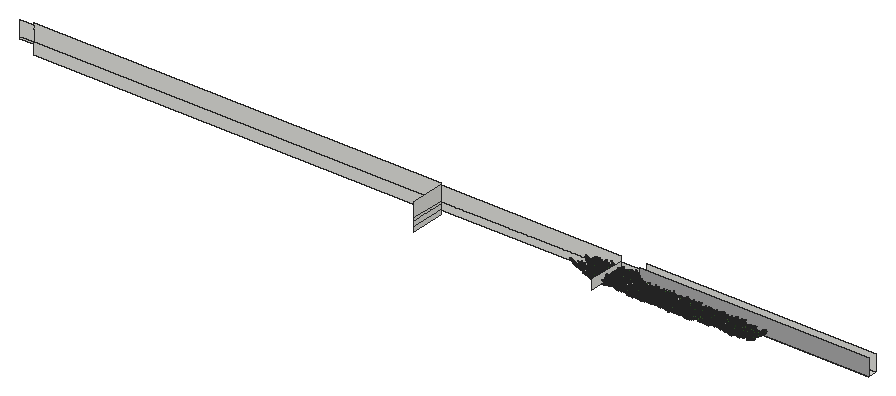
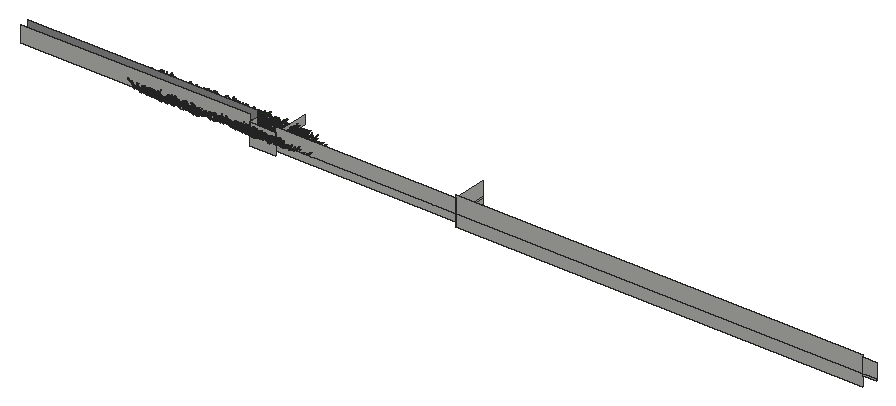
# SketchUp Ruby script. Lengths in inches.
U = 1.inch
M = Sketchup.active_model
def pt(a) = Geom::Point3d.new(a.map { |v| v * U })
def face(e, loops, mat)
  f = e.add_face(loops[0].map { |a| pt(a) })
  loops[1..].each { |l| e.add_face(l.map { |a| pt(a) }).erase! }
  f.material = f.back_material = mat if mat
  f
end
# faces: each face lists its corners as indices into pts; further lists are holes
def faces(e, pts, list, mat = nil) = list.each { |f| face(e, (f[0].is_a?(Array) ? f : [f]).map { |l| l.map { |i| pts[i] } }, mat) }
# xy, xz, yz: faces in a plane at the given z, y or x. An outline is a flat list of corners, or four numbers for a rectangle; further outlines are holes
def ring(l) = l.size == 4 ? [[l[0], l[1]], [l[2], l[1]], [l[2], l[3]], [l[0], l[3]]] : l.each_slice(2).to_a
def flat(e, list, mat, &to3) = list.each { |f| face(e, (f[0].is_a?(Array) ? f : [f]).map { |l| ring(l).map { |u, v| to3.(u, v) } }, mat) }
def xy(e, z, list, mat = nil) = flat(e, list, mat) { |x, y| [x, y, z] }
def xz(e, y, list, mat = nil) = flat(e, list, mat) { |x, z| [x, y, z] }
def yz(e, x, list, mat = nil) = flat(e, list, mat) { |y, z| [x, y, z] }
def lines(e, pts, list) = list.each { |a, b| e.add_line(pt(pts[a]), pt(pts[b])) }
# prism: a flat outline (further loops are holes) pulled along v
def prism(e, loops, v, mat = nil)
  f = face(e, loops, mat); d = Geom::Vector3d.new(v.map { |x| x * U })
  f.pushpull(f.normal.samedirection?(d) ? d.length : -d.length)
end
def box(e, o, s, mat = nil) = prism(e, [[o, [o[0] + s[0], o[1], o[2]], [o[0] + s[0], o[1] + s[1], o[2]], [o[0], o[1] + s[1], o[2]]]], [0, 0, s[2]], mat)
def at(x, y, z, deg = 0) = Geom::Transformation.translation(pt([x, y, z])) * Geom::Transformation.rotation(ORIGIN, Z_AXIS, deg.degrees)
def axes(o, x, y, z) = Geom::Transformation.new([*x, 0, *y, 0, *z, 0, *pt(o).to_a, 1])
def part(name) = M.definitions.add(name)
# library, detail: a bought-in or finely detailed component or shape, given as its bounding box
def library(name, o, s) = part(name).tap { |d| box(d.entities, o, s) }
def detail(e, o, s) = box(e.add_group.entities, o, s)
def put(e, d, t, mat = nil) = e.add_instance(d, t).tap { |i| i.material = mat if mat }
def group(e, t, mat = nil) = e.add_group.tap { |g| g.transformation = t; g.material = mat if mat }.entities
root = M.entities
M.materials.add("Material82").color = [68, 110, 58]
M.materials.add("Material83").color = [48, 90, 38]
M.materials.add("Material84").color = [68, 110, 48]
M.materials.add("Material85").color = [48, 90, 48]
M.materials.add("Material86").color = [58, 110, 58]
M.materials.add("Material87").color = [58, 90, 38]
M.materials.add("Material88").color = [68, 100, 58]
M.materials.add("Material89").color = [48, 100, 38]
M.materials.add("[Color M03]1").color = [170, 170, 170]
c1 = part("grass00")
p = [[-0.6875,0.15,0],[-0.56,0.08,5.52],[-0.04,0.03,2.76],[0.48,-0.02,0],[0.35,-0.02,5.52],[-0.1,-0.14,5.52],
  [-0.12,0.65,8.37],[-0.42,0.65,8.37]]
faces(c1.entities,p,[[0,1,2,3],[3,2,4],[1,5,2],[5,4,2],[1,6,5],[4,5,6],[7,6,1]])
c2 = part("Group16\#1")
put(c2.entities,c1,axes([1.44,-0.61,-0.01],[0.05352,0.12609,0],[-0.10704,0.04543,0.07239],[0.06664,-0.02828,0.11628]),"Material85")
put(c2.entities,c1,axes([0.76,-0.15,-0.01],[0.04676,0.24062,0],[-0.23162,0.04501,0.06642],[0.0652,-0.01267,0.23595]),"Material82")
put(c2.entities,c1,axes([0.79,0.01,-0.01],[-0.00606,0.34651,0],[-0.34381,-0.00602,0.0432],[0.04319,0.00076,0.34386]))
put(c2.entities,c1,axes([1,0.23,-0.01],[-0.07192,0.31144,0],[-0.28722,-0.06632,0.1236],[0.12043,0.02781,0.29478]),"Material84")
put(c2.entities,c1,axes([1.66,0.77,-0.01],[-0.13828,0.29651,0],[-0.21551,-0.1005,0.22471],[0.20365,0.09498,0.23779]),"Material89")
put(c2.entities,c1,axes([0.6875,0.52,-0.01],[-0.18126,0.24051,0],[-0.22746,-0.17142,0.09788],[0.07817,0.05891,0.28481]),"Material84")
put(c2.entities,c1,axes([0.68,0.78,-0.01],[-0.215,0.18688,0],[-0.12385,-0.14248,0.21334],[0.13995,0.16101,0.18878]),"Material82")
put(c2.entities,c1,axes([0.56,1,-0.01],[-0.13756,0.07624,0],[-0.06159,-0.11112,0.0927],[0.04494,0.08108,0.12705]),"Material84")
put(c2.entities,c1,axes([0.2,0.64,-0.01],[-0.23729,0.07254,0],[-0.05711,-0.18681,0.153],[0.04473,0.14632,0.19535]),"Material89")
put(c2.entities,c1,axes([0.0625,0.72,-0.01],[-0.28874,0.02525,0],[-0.02179,-0.24916,0.14647],[0.01276,0.14591,0.25012]),"Material82")
put(c2.entities,c1,axes([-0.08,0.62,-0.01],[-0.34089,-0.04187,0],[0.03255,-0.26504,0.216],[-0.02633,0.21439,0.26703]),"Material89")
put(c2.entities,c1,axes([-0.34,0.98,-0.01],[-0.14314,-0.0493,0],[0.04397,-0.12769,0.06843],[-0.02228,0.0647,0.13505]),"Material89")
put(c2.entities,c1,axes([-0.87,1.45,-0.01],[-0.23488,-0.14114,0],[0.13761,-0.22901,0.06087],[-0.03135,0.05217,0.26717]))
put(c2.entities,c1,axes([-0.72,0.77,-0.01],[-0.14208,-0.13251,0],[0.07209,-0.0773,0.16301],[-0.11118,0.11922,0.1057]),"Material89")
put(c2.entities,c1,axes([-0.62,0.43,-0.01],[-0.14845,-0.21203,0],[0.18654,-0.13061,0.12304],[-0.10079,0.07057,0.22772]),"Material82")
put(c2.entities,c1,axes([-0.68,0.29,-0.01],[-0.13639,-0.32136,0],[0.31723,-0.13464,0.05579],[-0.05136,0.0218,0.34462]),"Material83")
put(c2.entities,c1,axes([-0.64,0.125,-0.01],[-0.0458,-0.23569,0],[0.22124,-0.043,0.08276],[-0.08124,0.01579,0.22538]),"Material86")
put(c2.entities,c1,axes([-1.6,-0.03,-0.01],[0.00576,-0.32897,0],[0.27526,0.00482,0.18018],[-0.18015,-0.00315,0.2753]),"Material84")
put(c2.entities,c1,axes([-1.36,-0.31,-0.01],[0.05718,-0.24765,0],[0.18172,0.04196,0.17267],[-0.16825,-0.03885,0.1865]),"Material89")
put(c2.entities,c1,axes([-1.54,-0.72,-0.01],[0.06537,-0.14017,0],[0.13555,0.06321,0.03939],[-0.0357,-0.01665,0.14956]))
put(c2.entities,c1,axes([-1.19,-0.9,-0.01],[0.09597,-0.12735,0],[0.11214,0.08451,0.07557],[-0.06035,-0.04548,0.14042]),"Material88")
put(c2.entities,c1,axes([-0.47,-0.54,-0.01],[0.11588,-0.10072,0],[0.0618,0.0711,0.12124],[-0.07953,-0.0915,0.0942]))
put(c2.entities,c1,axes([-0.47,-0.84,-0.01],[0.11927,-0.0661,0],[0.06603,0.11913,0.00646],[-0.00313,-0.00565,0.13621]),"Material84")
put(c2.entities,c1,axes([-0.38,-1.24,-0.01],[0.28037,-0.08571,0],[0.0618,0.20215,0.20315],[-0.05939,-0.19428,0.21139]),"Material88")
put(c2.entities,c1,axes([-0.06,-0.66,-0.01],[0.22719,-0.01987,0],[0.01247,0.14255,0.17758],[-0.01547,-0.17691,0.1431]),"Material87")
put(c2.entities,c1,axes([0.11,-0.89,-0.01],[0.14882,0.01828,0],[-0.01058,0.08611,0.12229],[0.01491,-0.12138,0.08676]),"Material85")
put(c2.entities,c1,axes([0.25,-0.72,-0.01],[0.20481,0.07053,0],[-0.06206,0.18022,0.10291],[0.03351,-0.0973,0.1906]),"Material85")
put(c2.entities,c1,axes([0.85,-1.42,-0.01],[0.16481,0.09904,0],[-0.09472,0.15762,0.05616],[0.02893,-0.04814,0.18389]),"Material84")
put(c2.entities,c1,axes([1.01,-1.09,-0.01],[0.21858,0.20385,0],[-0.17495,0.1876,0.15339],[0.10462,-0.11218,0.25652]),"Material89")
put(c2.entities,c1,axes([1.01,-0.71,-0.01],[0.08733,0.12473,0],[-0.06445,0.04512,0.13037],[0.1068,-0.07477,0.07867]),"Material85")
c3 = part("Group15\#1")
put(c3.entities,c2,at(0,0,0))
c4 = part("3darcstudiotree_grass00\#1")
put(c4.entities,c3,at(0,0,0))
xy(root,-34.17,[[626.68,381.72,782.78,387.84]])
xz(root,381.72,[[626.68,-34.17,782.78,-22.8]],"[Color M03]1")
xz(root,387.84,[[208.91,-42.1875,486.41,-34.17],[609.09,-42.1875,626.68,-34.17],[486.41,-39.125,609.09,-34.17],[200.03,-35.625,208.91,-34.17],[200.03,-34.17,208.91,-24.25],
  [208.91,-34.17,486.41,-22.8],[486.41,-34.17,609.09,-24.25],[609.09,-34.17,626.68,-27.66],[626.68,-34.17,782.78,-22.8]])
yz(root,486.41,[[364.46,-42.1875,387.84,-39.125],[364.46,-39.125,387.84,-35.625],[364.46,-35.625,387.84,-34.17],[364.46,-34.17,387.84,-24.25]])
yz(root,609.09,[[362.97,-34.17,387.84,-27.66]])
yz(root,626.68,[[381.72,-34.17,387.84,-27.66]])
put(root,c4,axes([652.09,372.41,-34.17],[-4.26886,-0.01451,0],[0.03771,-1.72573,-0.00939],[0.00047,-0.02147,1.9024]))
put(root,c4,axes([641.22,372.79,-34.17],[3.91894,1.05311,0],[-2.36552,1.3691,-0.06012],[-0.14517,0.08402,1.3502]))
put(root,c4,axes([633.56,373.13,-34.17],[3.33812,-0.00931,0],[0.03014,1.68097,-0.0442],[0.00131,0.07293,1.33678]))
put(root,c4,axes([607.1,373.02,-34.17],[2.55431,1.01117,0],[-3.10398,1.2195,-0.03194],[-0.09397,0.03692,1.36388]))
put(root,c4,axes([664.3125,372.65,-34.17],[-3.78642,0.03695,0],[-0.11198,-1.78455,-0.01248],[-0.00125,-0.01991,1.37214]))
put(root,c4,axes([695.84,372.82,-34.17],[-3.59063,0.36551,0],[-0.927,-1.41632,-0.03018],[-0.05381,-0.08221,1.98332]))
put(root,c4,axes([668.4,372.76,-34.17],[-3.89357,0.61481,0],[-1.50479,-1.48217,-0.00598],[-0.01246,-0.01228,1.70205]))
put(root,c4,axes([631.51,373.3125,-34.17],[-2.43659,-1.39628,0],[3.54139,-0.96116,-0.05298],[0.19991,-0.05426,1.4759]))
put(root,c4,axes([622.52,373.45,-34.17],[2.25035,1.16277,0],[-2.68664,0.80868,-0.04536],[-0.27393,0.08245,1.92466]))
put(root,c4,axes([672.23,374.24,-34.17],[0.94723,-1.59052,0],[4.2139,0.39031,-0.04288],[0.2193,0.02031,1.70449]))
put(root,c4,axes([702.36,374.25,-34.17],[4.40385,0.48107,0],[-1.25638,1.78876,-0.02222],[-0.03253,0.04631,1.93436]))
put(root,c4,axes([664.33,374.63,-34.17],[0.52677,-1.54843,0],[3.37532,0.17859,-0.00096],[0.0064,0.00034,1.71349]))
put(root,c4,axes([607.1,374.65,-34.17],[1.00905,-1.48256,0],[4.12419,0.43657,-0.05256],[0.2523,0.02671,1.59089]))
put(root,c4,axes([669.5,374.45,-34.17],[-2.54975,-1.13663,0],[2.74994,-0.95943,-0.02762],[0.1264,-0.0441,1.68176]))
put(root,c4,axes([655.52,374.86,-34.17],[4.10302,-0.30694,0],[0.8385,1.74326,-0.00778],[0.00611,0.0127,1.42033]))
put(root,c4,axes([628.73,374.0625,-34.17],[-3.06856,1.30795,0],[-2.89535,-1.05647,-0.0352],[-0.142,-0.05181,1.62511]))
put(root,c4,axes([641.16,374.78,-34.17],[0.60137,-1.69863,0],[3.35822,0.18491,-0.0384],[0.22932,0.01263,1.53253]))
put(root,c4,axes([684.16,375.0625,-34.17],[3.06207,-0.55792,0],[1.42852,1.21938,-0.0238],[0.07482,0.06387,1.9133]))
put(root,c4,axes([679.29,374.52,-34.17],[0.41076,1.77313,0],[-3.60416,0.12986,-0.02215],[-0.11578,0.00417,1.42375]))
put(root,c4,axes([623.97,375.43,-34.17],[-0.12471,-1.80139,0],[4.72201,-0.05084,-0.06757],[0.3331,-0.00359,1.74608]))
put(root,c4,axes([633.75,374.875,-34.17],[-0.2328,1.40639,0],[-3.78045,-0.09733,-0.01044],[-0.05523,-0.00142,1.50484]))
put(root,c4,axes([695.93,374.77,-34.17],[-1.9685,1.46825,0],[-4.07305,-0.84931,-0.01892],[-0.07094,-0.01479,1.46501]))
put(root,c4,axes([613.67,375.07,-34.17],[1.86247,1.54763,0],[-3.42195,0.64048,-0.01135],[-0.06523,0.01221,1.80626]))
put(root,c4,axes([602.53,375.22,-34.17],[-0.22309,1.29668,0],[-4.38525,-0.11734,-0.00038],[-0.00168,-0.00004,1.44006]))
put(root,c4,axes([688.73,375.41,-34.17],[1.22817,1.22832,0],[-3.29828,0.51292,-0.04901],[-0.28268,0.04396,1.64754]))
put(root,c4,axes([649.625,375.32,-34.17],[-0.96459,1.39728,0],[-4.50708,-0.48391,-0.06593],[-0.29103,-0.03125,1.60187]))
put(root,c4,axes([647.97,375.42,-34.17],[0.06651,1.49398,0],[-4.62108,0.032,-0.00579],[-0.03066,0.00021,1.83497]))
put(root,c4,axes([616.87,375.59,-34.17],[-3.98386,-0.59662,0],[1.47731,-1.53422,-0.04397],[0.0965,-0.10022,1.92843]))
put(root,c4,axes([644.95,376.5,-34.17],[3.81628,-0.13918,0],[0.37321,1.59155,-0.00914],[0.00528,0.02252,1.90465]))
put(root,c4,axes([616.65,376.41,-34.17],[3.87274,-0.73751,0],[1.55178,1.26734,-0.04306],[0.13654,0.11151,1.95064]))
put(root,c4,axes([694.93,376.96,-34.17],[4.03419,0.29669,0],[-0.75311,1.59264,-0.00417],[-0.00465,0.00984,1.87295]))
put(root,c4,axes([657.29,376.69,-34.17],[1.8424,1.14237,0],[-3.65624,0.91712,-0.00074],[-0.00371,0.00093,1.93092]))
put(root,c4,axes([601.27,376.95,-34.17],[-2.10821,-1.47996,0],[3.50963,-0.77757,-0.0488],[0.18715,-0.04146,1.32723]))
put(root,c4,axes([690.03,376.96,-34.17],[4.26727,0.66803,0],[-1.41698,1.40776,-0.04113],[-0.07249,0.07202,1.37498]))
put(root,c4,axes([672.39,377.2,-34.17],[4.15464,-0.59094,0],[1.53872,1.68251,-0.06016],[0.09162,0.10018,1.52593]))
put(root,c4,axes([668.37,376.61,-34.17],[0.64746,1.71828,0],[-3.59,0.21039,-0.03328],[-0.18561,0.01088,1.53387]))
put(root,c4,axes([606.1,377.25,-34.17],[2.13524,-1.29449,0],[3.0122,0.77275,-0.01966],[0.10051,0.02579,1.64285]))
put(root,c4,axes([641.33,376.78,-34.17],[-1.5249,1.25696,0],[-3.62628,-0.68422,-0.02774],[-0.1175,-0.02217,1.41462]))
put(root,c4,axes([623.77,377.47,-34.17],[3.32502,-0.81851,0],[2.11953,1.33913,-0.03499],[0.11667,0.07371,1.88939]))
put(root,c4,axes([597.38,376.76,-34.17],[-3.35215,0.96429,0],[-2.54913,-1.37823,-0.03459],[-0.11585,-0.06264,1.84283]))
put(root,c4,axes([661.1,377.42,-34.17],[-1.38876,-1.54798,0],[3.56891,-0.49797,-0.03351],[0.18812,-0.02625,1.68972]))
put(root,c4,axes([634.32,376.83,-34.17],[-1.7842,1.38137,0],[-4.14651,-0.83297,-0.01882],[-0.07173,-0.01441,1.49212]))
put(root,c4,axes([680.47,377.7,-34.17],[0.96466,-1.81909,0],[3.32191,0.27398,-0.01603],[0.09156,0.00755,1.48463]))
put(root,c4,axes([614.5,377.27,-34.17],[-2.42169,0.94143,0],[-3.12641,-1.2508,-0.05994],[-0.19111,-0.07646,1.51606]))
put(root,c4,axes([627.52,377.69,-34.17],[-1.63198,-1.29559,0],[3.66951,-0.7189,-0.01655],[0.08632,-0.01691,1.78815]))
put(root,c4,axes([686.3,377.29,-34.17],[-1.97144,1.08801,0],[-3.33394,-0.93955,-0.01309],[-0.05439,-0.01533,1.56859]))
put(root,c4,axes([701.74,377.8,-34.17],[-3.77025,-0.95024,0],[2.35793,-1.45505,-0.05584],[0.17762,-0.10961,1.93872]))
put(root,c4,axes([652.15,377.51,-34.17],[-0.60649,1.78928,0],[-3.60415,-0.19,-0.04319],[-0.29403,-0.0155,1.87209]))
put(root,c4,axes([668.95,378.77,-34.17],[2.12492,-1.52639,0],[3.32667,0.72027,-0.02765],[0.13101,0.02837,1.53783]))
put(root,c4,axes([597.24,378.7,-34.17],[3.10066,0.47843,0],[-1.67535,1.68868,-0.03882],[-0.06401,0.06452,1.55956]))
put(root,c4,axes([602.84,378.47,-34.17],[2.78968,1.01154,0],[-2.64,1.13236,-0.04265],[-0.18761,0.08047,1.90027]))
put(root,c4,axes([612.4,378.8,-34.17],[4.11116,0.47333,0],[-1.05643,1.42708,-0.03197],[-0.04362,0.05892,1.37583]))
put(root,c4,axes([640.57,378.72,-34.17],[3.33503,1.17525,0],[-2.6851,1.18507,-0.00121],[-0.00399,0.00176,1.48985]))
put(root,c4,axes([674.12,379.08,-34.17],[2.11135,-1.17998,0],[3.12805,0.87051,-0.01427],[0.05324,0.01482,1.30992]))
put(root,c4,axes([658.07,379,-34.17],[-2.24585,-1.17679,0],[2.75058,-0.81643,-0.02546],[0.1532,-0.04547,1.94365]))
put(root,c4,axes([679.77,379.3,-34.17],[-1.90322,-1.23489,0],[2.93996,-0.70472,-0.04312],[0.27444,-0.06578,1.92045]))
put(root,c4,axes([606.78,378.9,-34.17],[-2.52665,1.52426,0],[-3.1276,-0.80632,-0.05029],[-0.29899,-0.07708,1.98932]))
put(root,c4,axes([651.6,378.94,-34.17],[-1.50368,1.17097,0],[-3.52829,-0.70467,-0.03106],[-0.12382,-0.02473,1.32443]))
put(root,c4,axes([700.05,379.75,-34.17],[3.38929,-0.88137,0],[2.3631,1.41334,-0.02666],[0.06787,0.04059,1.48784]))
put(root,c4,axes([663.3125,379.73,-34.17],[2.20658,-1.37183,0],[2.86337,0.71632,-0.01781],[0.08885,0.02223,1.50117]))
put(root,c4,axes([645,379.64,-34.17],[0.14571,-1.35454,0],[4.55175,0.07615,-0.04061],[0.20314,0.0034,1.70991]))
put(root,c4,axes([690.06,379.53,-34.17],[3.73542,0.56333,0],[-1.36375,1.40645,-0.02441],[-0.06005,0.06193,1.97124]))
put(root,c4,axes([617.67,379.17,-34.17],[0.11998,1.39847,0],[-4.49149,0.05993,-0.06181],[-0.32467,0.00433,1.77032]))
put(root,c4,axes([685.36,379.47,-34.17],[2.76774,0.7917,0],[-1.93345,1.05126,-0.02439],[-0.09329,0.05072,1.60766]))
put(root,c4,axes([623.83,379.76,-34.17],[2.90846,1.13793,0],[-2.61613,1.03996,-0.02475],[-0.10205,0.04057,1.62992]))
put(root,c4,axes([695.87,379.87,-34.17],[1.66114,1.62878,0],[-3.87747,0.61504,-0.0015],[-0.00686,0.00109,1.54039]))
put(root,c4,axes([627.625,379.91,-34.17],[0.65055,1.72425,0],[-3.43127,0.20135,-0.01524],[-0.11013,0.00646,1.90022]))
put(root,c4,axes([636.29,379.91,-34.17],[-2.50108,0.95556,0],[-2.98511,-1.21518,-0.02879],[-0.10959,-0.04461,1.7592]))
put(root,c4,axes([688.81,380.69,-34.17],[2.03121,-1.05332,0],[3.7313,1.11909,-0.04371],[0.13933,0.04179,1.40723]))
put(root,c4,axes([623.9375,380.76,-34.17],[4.3644,0.14123,0],[-0.27589,1.32601,-0.01884],[-0.00836,0.04017,1.37151]))
put(root,c4,axes([607.96,380.67,-34.17],[4.04964,0.85012,0],[-2.04869,1.51784,-0.02998],[-0.08539,0.06326,1.98098]))
put(root,c4,axes([633.9375,380.75,-34.17],[-0.81871,-1.45227,0],[3.80429,-0.33355,-0.01455],[0.06635,-0.00582,1.36448]))
put(root,c4,axes([669.2,381.01,-34.17],[2.26224,-1.2031,0],[3.43735,1.00525,-0.03781],[0.13632,0.03987,1.4396]))
put(root,c4,axes([653.54,381.18,-34.17],[3.40778,-1.13854,0],[2.78991,1.29874,-0.02128],[0.06823,0.03176,1.60475]))
put(root,c4,axes([673.07,380.76,-34.17],[-4.28344,0.1007,0],[-0.25434,-1.68266,-0.00226],[-0.00079,-0.00521,1.87745]))
put(root,c4,axes([702.07,380.75,-34.17],[-3.53825,1.08299,0],[-2.59336,-1.31776,-0.03049],[-0.10241,-0.05204,1.73706]))
put(root,c4,axes([611.7,381.41,-34.17],[3.8777,-0.38352,0],[0.80355,1.2636,-0.03452],[0.06321,0.0994,1.86367]))
put(root,c4,axes([694.64,381.04,-34.17],[-3.68784,-0.24252,0],[0.55953,-1.32329,-0.01602],[0.01459,-0.0345,1.41148]))
put(root,c4,axes([602.6,381.09,-34.17],[-3.74626,-0.28421,0],[0.67953,-1.39309,-0.01319],[0.01627,-0.03336,1.76124]))
put(root,c4,axes([658.01,381.61,-34.17],[1.48309,-1.18944,0],[3.17184,0.61511,-0.04022],[0.27217,0.05278,1.99791]))
put(root,c4,axes([683.51,381.65,-34.17],[3.41982,0.22152,0],[-0.58321,1.40029,-0.00501],[-0.00425,0.0102,1.40942]))
put(root,c4,axes([616.94,381.62,-34.17],[3.19951,0.37191,0],[-1.24549,1.66647,-0.04213],[-0.05146,0.06886,1.42653]))
put(root,c4,axes([631.55,381.27,-34.17],[1.18703,1.24458,0],[-3.56072,0.52819,-0.04913],[-0.2933,0.04351,1.81865]))
put(root,c4,axes([639.32,381.82,-34.17],[4.2261,-0.33522,0],[0.81524,1.59847,-0.02659],[0.0257,0.05039,1.51897]))
put(root,c4,axes([664.82,381.11,-34.17],[-4.05008,0.95977,0],[-1.76425,-1.15789,-0.02116],[-0.06339,-0.0416,1.49339]))
put(root,c4,axes([677.88,381.27,-34.17],[-2.75564,1.16599,0],[-3.11928,-1.14656,-0.00031],[-0.00116,-0.00043,1.61707]))
put(root,c4,axes([646.06,382.22,-34.17],[-4.64372,0.01964,0],[-0.04703,-1.72937,-0.01941],[-0.00122,-0.04491,1.92834]))
put(root,c4,axes([622.42,382.97,-34.17],[1.86264,-1.28665,0],[3.53883,0.79678,-0.00497],[0.01917,0.00432,1.35772]))
put(root,c4,axes([636.12,383.25,-34.17],[0.27542,-1.59187,0],[4.66457,0.12552,-0.02398],[0.0893,0.0024,1.30813]))
put(root,c4,axes([628.68,382.93,-34.17],[-3.57616,-1.16474,0],[2.7999,-1.33704,-0.02974],[0.0776,-0.03706,1.35064]))
put(root,c4,axes([658.92,383.33,-34.17],[-1.75334,-1.53625,0],[3.78301,-0.67151,-0.04331],[0.23983,-0.04257,1.88835]))
put(root,c4,axes([688.45,383.01,-34.17],[-3.93222,-0.02635,0],[0.07503,-1.74154,-0.03595],[0.00307,-0.07126,1.66434]))
put(root,c4,axes([598.4,383.51,-34.17],[-1.52778,-1.4368,0],[3.26203,-0.53947,-0.00949],[0.054,-0.00893,1.63563]))
put(root,c4,axes([607.54,383.58,-34.17],[-0.81771,-1.39799,0],[3.86882,-0.35195,-0.03351],[0.1754,-0.01596,1.59864]))
put(root,c4,axes([686.62,383.74,-34.17],[1.79387,-1.26785,0],[3.18419,0.70071,-0.05199],[0.23586,0.0519,1.41973]))
put(root,c4,axes([663.72,383.7,-34.17],[-0.47275,-1.4969,0],[4.46074,-0.21911,-0.06365],[0.35527,-0.01745,1.89522]))
put(root,c4,axes([646.04,383.84,-34.17],[4.39151,-0.30239,0],[0.81207,1.8342,-0.04063],[0.02885,0.06516,1.46079]))
put(root,c4,axes([640,383.8,-34.17],[0.23544,-1.60034,0],[3.90526,0.08936,-0.02273],[0.11635,0.00266,1.50351]))
put(root,c4,axes([619.98,383.68,-34.17],[4.04452,0.28903,0],[-0.72611,1.58031,-0.0513],[-0.04641,0.10101,1.54883]))
put(root,c4,axes([697.66,383.49,-34.17],[-2.90199,-1.04001,0],[2.97522,-1.29119,-0.02206],[0.0727,-0.03155,1.62457]))
put(root,c4,axes([678.23,383.9375,-34.17],[-0.12409,-1.44715,0],[3.33282,-0.04445,-0.02047],[0.13634,-0.00182,1.66543]))
put(root,c4,axes([651.74,384.15,-34.17],[2.16016,-1.57069,0],[3.42867,0.73339,-0.01711],[0.07383,0.01579,1.43496]))
put(root,c4,axes([602.25,383.9375,-34.17],[-1.12016,-1.49158,0],[3.32126,-0.38792,-0.01669],[0.11216,-0.0131,1.82011]))
put(root,c4,axes([673.93,383.7,-34.17],[0.32393,1.2922,0],[-3.8703,0.1509,-0.01511],[-0.10076,0.00393,1.95375]))
put(root,c4,axes([613.75,384.33,-34.17],[3.3382,-1.0215,0],[2.0281,1.0308,-0.00126],[0.00417,0.00212,1.3431]))
put(root,c4,axes([668.45,384.13,-34.17],[-3.07387,-1.37226,0],[2.57369,-0.89663,-0.00245],[0.01347,-0.00469,1.8862]))
put(root,c4,axes([702.84,384.2,-34.17],[1.42863,1.44478,0],[-4.37041,0.67213,-0.01645],[-0.07678,0.01181,1.76201]))
put(root,c4,axes([614.47,385.08,-34.17],[1.09339,-1.57965,0],[4.13626,0.44528,-0.00598],[0.02433,0.00262,1.35627]))
put(root,c4,axes([695.82,385.23,-34.17],[1.06749,-1.46896,0],[3.76494,0.42553,-0.03571],[0.22932,0.02592,1.9611]))
put(root,c4,axes([629.17,385.49,-34.17],[3.96997,0.02835,0],[-0.08063,1.7564,-0.04973],[-0.00512,0.11159,1.89995]))
put(root,c4,axes([690.54,385.27,-34.17],[1.59793,1.26945,0],[-3.48077,0.68144,-0.01001],[-0.04528,0.00886,1.4706]))
put(root,c4,axes([634.52,385.48,-34.17],[-3.18032,-1.25414,0],[2.9494,-1.16324,-0.05204],[0.20858,-0.08226,1.77215]))
put(root,c4,axes([640.12,385.59,-34.17],[3.671,0.98063,0],[-2.61565,1.5229,-0.02464],[-0.07837,0.04563,1.98292]))
put(root,c4,axes([672.74,385.83,-34.17],[1.6756,-1.36696,0],[3.5262,0.67226,-0.03335],[0.16368,0.0312,1.60043]))
put(root,c4,axes([644.625,386.03,-34.17],[3.22571,-1.00591,0],[2.69072,1.34198,-0.01988],[0.07446,0.03714,1.96304]))
put(root,c4,axes([702.34,386.04,-34.17],[2.00503,-1.14609,0],[3.00042,0.81639,-0.0362],[0.21042,0.05725,1.92943]))
put(root,c4,axes([659.07,385.98,-34.17],[-1.47837,-1.71881,0],[3.4357,-0.4596,-0.01224],[0.08437,-0.01129,1.97883]))
put(root,c4,axes([666.75,386.02,-34.17],[-0.70107,-1.67232,0],[4.13597,-0.26967,-0.0168],[0.0818,-0.00533,1.55067]))
put(root,c4,axes([606.72,385.5,-34.17],[-2.75278,0.82906,0],[-2.65464,-1.37089,-0.0597],[-0.21369,-0.11035,1.93343]))
put(root,c4,axes([617.62,385.77,-34.17],[3.04278,1.18912,0],[-3.29647,1.31191,-0.05903],[-0.21773,0.08665,1.83956]))
put(root,c4,axes([597.35,385.77,-34.17],[-2.50316,1.24796,0],[-3.26881,-1.01974,-0.0328],[-0.10917,-0.03406,1.32564]))
put(root,c4,axes([622.72,386.54,-34.17],[2.18615,-1.3842,0],[3.44906,0.84721,-0.04551],[0.21226,0.05214,1.67334]))
put(root,c4,axes([600.85,386.22,-34.17],[-3.58141,-0.41852,0],[1.07572,-1.43168,-0.05017],[0.07746,-0.10309,1.54202]))
put(root,c4,axes([664.53,386.12,-34.17],[-3.50363,0.54877,0],[-1.37004,-1.36042,-0.04199],[-0.09387,-0.09321,1.68502]))
put(root,c4,axes([679.1,386.18,-34.17],[1.45904,1.69634,0],[-4.12454,0.55175,-0.04327],[-0.22093,0.02955,1.7601]))
put(root,c4,axes([650.99,386.58,-34.17],[-1.03876,-1.58927,0],[3.98467,-0.40506,-0.01269],[0.06748,-0.00686,1.69312]))
put(root,c4,axes([685.61,386.55,-34.17],[3.16719,1.22877,0],[-2.37702,0.9529,-0.00671],[-0.02839,0.01138,1.53359]))
put(root,c4,axes([613.58,387.62,-34.17],[3.59653,-0.21085,0],[0.631,1.67397,-0.00967],[0.00626,0.01661,1.41667]))
put(root,c4,axes([667.32,387.57,-34.17],[3.86987,-0.34459,0],[0.79622,1.39073,-0.03599],[0.03867,0.06754,1.32194]))
put(root,c4,axes([628.24,387.45,-34.17],[2.6716,0.78375,0],[-2.01413,1.06781,-0.0148],[-0.06741,0.03574,1.93047]))
put(root,c4,axes([696.34,387.2,-34.17],[-3.48173,-0.56284,0],[1.61416,-1.55298,-0.01809],[0.03189,-0.03068,1.4829]))
put(root,c4,axes([661.72,387.67,-34.17],[-0.94917,-1.78727,0],[4.28932,-0.35429,-0.02019],[0.10216,-0.00844,1.69814]))
put(root,c4,axes([603.15,387.42,-34.17],[-4.08051,-0.34509,0],[0.80518,-1.48079,-0.03168],[0.03378,-0.06213,1.46389]))
put(root,c4,axes([673,388.1,-34.17],[4.59121,-0.45029,0],[0.84969,1.34743,-0.00031],[0.00049,0.00078,1.72722]))
put(root,c4,axes([689.82,387.73,-34.17],[-2.98813,-0.54786,0],[1.47052,-1.24742,-0.04575],[0.11826,-0.10032,1.60296]))
put(root,c4,axes([620.27,387.875,-34.17],[-3.23469,-1.08731,0],[2.23739,-1.03522,-0.02002],[0.06548,-0.0303,1.30322]))
put(root,c4,axes([633.19,387.7,-34.17],[-4.17606,0.09309,0],[-0.21865,-1.52546,-0.00256],[-0.00085,-0.00591,1.70382]))
put(root,c4,axes([624.32,388.31,-34.17],[0.26998,-1.38938,0],[4.08981,0.1236,-0.05496],[0.34231,0.01035,1.9204]))
put(root,c4,axes([682.98,387.97,-34.17],[-3.32048,-0.89448,0],[2.67505,-1.54445,-0.03279],[0.08824,-0.05095,1.69581]))
